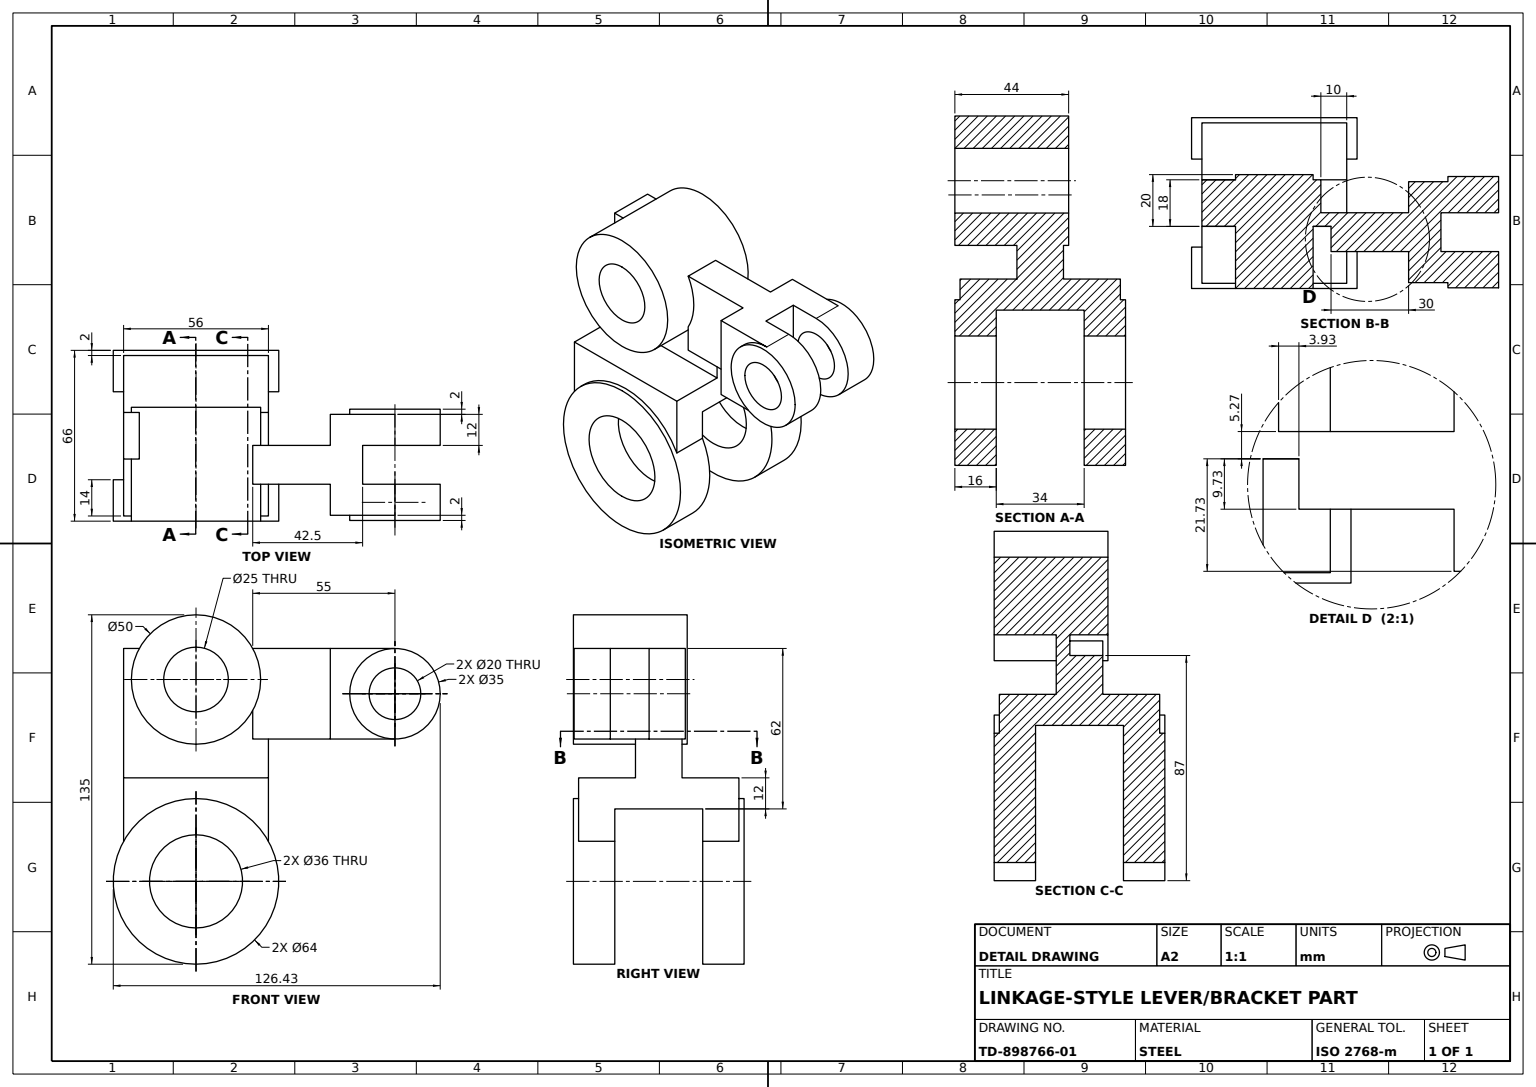
ISO-10303-21;
HEADER;
FILE_DESCRIPTION((''),'2;1');
FILE_NAME('','',(''),(''),'','','');
FILE_SCHEMA(('AUTOMOTIVE_DESIGN'));
ENDSEC;
DATA;
#1=APPLICATION_CONTEXT('');
#2=PRODUCT_CONTEXT('',#1,'mechanical');
#3=PRODUCT('','','',(#2));
#4=PRODUCT_DEFINITION_FORMATION('','',#3);
#5=PRODUCT_DEFINITION_CONTEXT('',#1,'design');
#6=PRODUCT_DEFINITION('','',#4,#5);
#7=PRODUCT_DEFINITION_SHAPE('','',#6);
#8=(LENGTH_UNIT()NAMED_UNIT(*)SI_UNIT(.MILLI.,.METRE.));
#9=(NAMED_UNIT(*)PLANE_ANGLE_UNIT()SI_UNIT($,.RADIAN.));
#10=(NAMED_UNIT(*)SI_UNIT($,.STERADIAN.)SOLID_ANGLE_UNIT());
#11=UNCERTAINTY_MEASURE_WITH_UNIT(LENGTH_MEASURE(1.E-05),#8,'distance_accuracy_value','');
#12=(GEOMETRIC_REPRESENTATION_CONTEXT(3)GLOBAL_UNCERTAINTY_ASSIGNED_CONTEXT((#11))GLOBAL_UNIT_ASSIGNED_CONTEXT((#8,#9,#10))REPRESENTATION_CONTEXT('',''));
#13=CARTESIAN_POINT('',(17.,-60.,-28.));
#14=VERTEX_POINT('',#13);
#15=CARTESIAN_POINT('',(17.,-12.508067,-56.));
#16=VERTEX_POINT('',#15);
#17=CARTESIAN_POINT('',(17.,-28.,-28.));
#18=DIRECTION('',(1.,0.,0.));
#19=DIRECTION('',(0.,1.,0.));
#20=AXIS2_PLACEMENT_3D('',#17,#18,#19);
#21=CIRCLE('',#20,32.);
#22=EDGE_CURVE('',#14,#16,#21,.T.);
#23=ORIENTED_EDGE('',*,*,#22,.T.);
#24=CARTESIAN_POINT('',(31.,-12.508067,-56.));
#25=VERTEX_POINT('',#24);
#26=DIRECTION('',(-1.,0.,0.));
#27=VECTOR('',#26,1000.);
#28=LINE('',#15,#27);
#29=EDGE_CURVE('',#25,#16,#28,.T.);
#30=ORIENTED_EDGE('',*,*,#29,.F.);
#31=CARTESIAN_POINT('',(31.,4.,-28.));
#32=VERTEX_POINT('',#31);
#33=CARTESIAN_POINT('',(31.,-28.,-28.));
#34=AXIS2_PLACEMENT_3D('',#33,#18,#19);
#35=CIRCLE('',#34,32.);
#36=EDGE_CURVE('',#25,#32,#35,.T.);
#37=ORIENTED_EDGE('',*,*,#36,.T.);
#38=CARTESIAN_POINT('',(33.,4.,-28.));
#39=VERTEX_POINT('',#38);
#40=CARTESIAN_POINT('',(17.,4.,-28.));
#41=VECTOR('',#18,1000.);
#42=LINE('',#40,#41);
#43=EDGE_CURVE('',#32,#39,#42,.T.);
#44=ORIENTED_EDGE('',*,*,#43,.T.);
#45=CARTESIAN_POINT('',(33.,-60.,-28.));
#46=VERTEX_POINT('',#45);
#47=CARTESIAN_POINT('',(33.,-28.,-28.));
#48=AXIS2_PLACEMENT_3D('',#47,#18,#19);
#49=CIRCLE('',#48,32.);
#50=EDGE_CURVE('',#46,#39,#49,.T.);
#51=ORIENTED_EDGE('',*,*,#50,.F.);
#52=LINE('',#13,#41);
#53=EDGE_CURVE('',#14,#46,#52,.T.);
#54=ORIENTED_EDGE('',*,*,#53,.F.);
#55=EDGE_LOOP('',(#23,#30,#37,#44,#51,#54));
#56=FACE_OUTER_BOUND('',#55,.T.);
#57=CYLINDRICAL_SURFACE('',#20,32.);
#58=ADVANCED_FACE('',(#56),#57,.T.);
#59=CARTESIAN_POINT('',(-17.,0.,0.));
#60=VERTEX_POINT('',#59);
#61=CARTESIAN_POINT('',(17.,0.,0.));
#62=VERTEX_POINT('',#61);
#63=CARTESIAN_POINT('',(0.,0.,0.));
#64=LINE('',#63,#41);
#65=EDGE_CURVE('',#60,#62,#64,.T.);
#66=ORIENTED_EDGE('',*,*,#65,.F.);
#67=CARTESIAN_POINT('',(-17.,0.,-56.));
#68=VERTEX_POINT('',#67);
#69=DIRECTION('',(0.,0.,1.));
#70=VECTOR('',#69,1000.);
#71=LINE('',#67,#70);
#72=EDGE_CURVE('',#68,#60,#71,.T.);
#73=ORIENTED_EDGE('',*,*,#72,.F.);
#74=CARTESIAN_POINT('',(17.,0.,-56.));
#75=VERTEX_POINT('',#74);
#76=CARTESIAN_POINT('',(0.,0.,-56.));
#77=LINE('',#76,#41);
#78=EDGE_CURVE('',#68,#75,#77,.T.);
#79=ORIENTED_EDGE('',*,*,#78,.T.);
#80=LINE('',#74,#70);
#81=EDGE_CURVE('',#75,#62,#80,.T.);
#82=ORIENTED_EDGE('',*,*,#81,.T.);
#83=EDGE_LOOP('',(#66,#73,#79,#82));
#84=FACE_OUTER_BOUND('',#83,.T.);
#85=DIRECTION('',(0.,-1.,0.));
#86=DIRECTION('',(0.,0.,-1.));
#87=AXIS2_PLACEMENT_3D('',#76,#85,#86);
#88=PLANE('',#87);
#89=ADVANCED_FACE('',(#84),#88,.T.);
#90=CARTESIAN_POINT('',(3.731987,27.,-104.931712));
#91=VERTEX_POINT('',#90);
#92=CARTESIAN_POINT('',(-8.268013,27.,-104.931712));
#93=VERTEX_POINT('',#92);
#94=LINE('',#92,#27);
#95=EDGE_CURVE('',#91,#93,#94,.T.);
#96=ORIENTED_EDGE('',*,*,#95,.F.);
#97=CARTESIAN_POINT('',(3.731987,27.,-92.431712));
#98=VERTEX_POINT('',#97);
#99=VECTOR('',#86,1000.);
#100=LINE('',#90,#99);
#101=EDGE_CURVE('',#98,#91,#100,.T.);
#102=ORIENTED_EDGE('',*,*,#101,.F.);
#103=CARTESIAN_POINT('',(18.731987,27.,-92.431712));
#104=VERTEX_POINT('',#103);
#105=LINE('',#97,#27);
#106=EDGE_CURVE('',#104,#98,#105,.T.);
#107=ORIENTED_EDGE('',*,*,#106,.F.);
#108=CARTESIAN_POINT('',(18.731987,27.,-104.931712));
#109=VERTEX_POINT('',#108);
#110=LINE('',#103,#70);
#111=EDGE_CURVE('',#109,#104,#110,.T.);
#112=ORIENTED_EDGE('',*,*,#111,.F.);
#113=CARTESIAN_POINT('',(30.731987,27.,-104.931712));
#114=VERTEX_POINT('',#113);
#115=LINE('',#108,#27);
#116=EDGE_CURVE('',#114,#109,#115,.T.);
#117=ORIENTED_EDGE('',*,*,#116,.F.);
#118=CARTESIAN_POINT('',(30.731987,27.,-79.931712));
#119=VERTEX_POINT('',#118);
#120=LINE('',#113,#99);
#121=EDGE_CURVE('',#119,#114,#120,.T.);
#122=ORIENTED_EDGE('',*,*,#121,.F.);
#123=CARTESIAN_POINT('',(18.731987,27.,-79.931712));
#124=VERTEX_POINT('',#123);
#125=LINE('',#118,#41);
#126=EDGE_CURVE('',#124,#119,#125,.T.);
#127=ORIENTED_EDGE('',*,*,#126,.F.);
#128=CARTESIAN_POINT('',(18.731987,27.,-49.931712));
#129=VERTEX_POINT('',#128);
#130=LINE('',#123,#99);
#131=EDGE_CURVE('',#129,#124,#130,.T.);
#132=ORIENTED_EDGE('',*,*,#131,.F.);
#133=CARTESIAN_POINT('',(9.,27.,-49.931712));
#134=VERTEX_POINT('',#133);
#135=CARTESIAN_POINT('',(3.731987,27.,-49.931712));
#136=LINE('',#135,#41);
#137=EDGE_CURVE('',#134,#129,#136,.T.);
#138=ORIENTED_EDGE('',*,*,#137,.F.);
#139=CARTESIAN_POINT('',(9.,27.,-56.));
#140=VERTEX_POINT('',#139);
#141=LINE('',#139,#99);
#142=EDGE_CURVE('',#134,#140,#141,.T.);
#143=ORIENTED_EDGE('',*,*,#142,.T.);
#144=CARTESIAN_POINT('',(3.731987,27.,-56.));
#145=VERTEX_POINT('',#144);
#146=CARTESIAN_POINT('',(0.,27.,-56.));
#147=LINE('',#146,#41);
#148=EDGE_CURVE('',#145,#140,#147,.T.);
#149=ORIENTED_EDGE('',*,*,#148,.F.);
#150=CARTESIAN_POINT('',(3.731987,27.,-79.931712));
#151=VERTEX_POINT('',#150);
#152=LINE('',#135,#70);
#153=EDGE_CURVE('',#151,#145,#152,.T.);
#154=ORIENTED_EDGE('',*,*,#153,.F.);
#155=CARTESIAN_POINT('',(-8.268013,27.,-79.931712));
#156=VERTEX_POINT('',#155);
#157=LINE('',#150,#41);
#158=EDGE_CURVE('',#156,#151,#157,.T.);
#159=ORIENTED_EDGE('',*,*,#158,.F.);
#160=LINE('',#155,#70);
#161=EDGE_CURVE('',#93,#156,#160,.T.);
#162=ORIENTED_EDGE('',*,*,#161,.F.);
#163=EDGE_LOOP('',(#96,#102,#107,#112,#117,#122,#127,#132,#138,#143,#149,#154,#159,#162));
#164=FACE_OUTER_BOUND('',#163,.T.);
#165=CARTESIAN_POINT('',(0.,27.,0.));
#166=AXIS2_PLACEMENT_3D('',#165,#85,#86);
#167=PLANE('',#166);
#168=ADVANCED_FACE('',(#164),#167,.T.);
#169=CARTESIAN_POINT('',(18.731987,38.,-49.931712));
#170=VERTEX_POINT('',#169);
#171=CARTESIAN_POINT('',(18.731987,62.,-49.931712));
#172=VERTEX_POINT('',#171);
#173=CARTESIAN_POINT('',(18.731987,50.,-28.));
#174=AXIS2_PLACEMENT_3D('',#173,#18,#86);
#175=CIRCLE('',#174,25.);
#176=EDGE_CURVE('',#170,#172,#175,.T.);
#177=ORIENTED_EDGE('',*,*,#176,.F.);
#178=VECTOR('',#19,1000.);
#179=LINE('',#128,#178);
#180=EDGE_CURVE('',#129,#170,#179,.T.);
#181=ORIENTED_EDGE('',*,*,#180,.F.);
#182=ORIENTED_EDGE('',*,*,#131,.T.);
#183=CARTESIAN_POINT('',(18.731987,62.,-79.931712));
#184=VERTEX_POINT('',#183);
#185=LINE('',#123,#178);
#186=EDGE_CURVE('',#124,#184,#185,.T.);
#187=ORIENTED_EDGE('',*,*,#186,.T.);
#188=LINE('',#183,#99);
#189=EDGE_CURVE('',#172,#184,#188,.T.);
#190=ORIENTED_EDGE('',*,*,#189,.F.);
#191=EDGE_LOOP('',(#177,#181,#182,#187,#190));
#192=FACE_OUTER_BOUND('',#191,.T.);
#193=AXIS2_PLACEMENT_3D('',#123,#18,#86);
#194=PLANE('',#193);
#195=ADVANCED_FACE('',(#192),#194,.T.);
#196=CARTESIAN_POINT('',(32.731987,44.5,-122.431712));
#197=VERTEX_POINT('',#196);
#198=CARTESIAN_POINT('',(18.731987,44.5,-122.431712));
#199=VERTEX_POINT('',#198);
#200=LINE('',#196,#27);
#201=EDGE_CURVE('',#197,#199,#200,.T.);
#202=ORIENTED_EDGE('',*,*,#201,.T.);
#203=CARTESIAN_POINT('',(18.731987,62.,-104.931712));
#204=VERTEX_POINT('',#203);
#205=CARTESIAN_POINT('',(18.731987,44.5,-104.931712));
#206=AXIS2_PLACEMENT_3D('',#205,#18,#86);
#207=CIRCLE('',#206,17.5);
#208=EDGE_CURVE('',#199,#204,#207,.T.);
#209=ORIENTED_EDGE('',*,*,#208,.T.);
#210=CARTESIAN_POINT('',(30.731987,62.,-104.931712));
#211=VERTEX_POINT('',#210);
#212=LINE('',#203,#27);
#213=EDGE_CURVE('',#211,#204,#212,.T.);
#214=ORIENTED_EDGE('',*,*,#213,.F.);
#215=CARTESIAN_POINT('',(30.731987,44.5,-87.431712));
#216=VERTEX_POINT('',#215);
#217=CARTESIAN_POINT('',(30.731987,44.5,-104.931712));
#218=AXIS2_PLACEMENT_3D('',#217,#18,#86);
#219=CIRCLE('',#218,17.5);
#220=EDGE_CURVE('',#211,#216,#219,.T.);
#221=ORIENTED_EDGE('',*,*,#220,.T.);
#222=CARTESIAN_POINT('',(32.731987,44.5,-87.431712));
#223=VERTEX_POINT('',#222);
#224=LINE('',#222,#27);
#225=EDGE_CURVE('',#223,#216,#224,.T.);
#226=ORIENTED_EDGE('',*,*,#225,.F.);
#227=CARTESIAN_POINT('',(32.731987,44.5,-104.931712));
#228=AXIS2_PLACEMENT_3D('',#227,#18,#86);
#229=CIRCLE('',#228,17.5);
#230=EDGE_CURVE('',#197,#223,#229,.T.);
#231=ORIENTED_EDGE('',*,*,#230,.F.);
#232=EDGE_LOOP('',(#202,#209,#214,#221,#226,#231));
#233=FACE_OUTER_BOUND('',#232,.T.);
#234=AXIS2_PLACEMENT_3D('',#227,#26,#69);
#235=CYLINDRICAL_SURFACE('',#234,17.5);
#236=ADVANCED_FACE('',(#233),#235,.T.);
#237=CARTESIAN_POINT('',(9.,62.,-6.068288));
#238=VERTEX_POINT('',#237);
#239=CARTESIAN_POINT('',(9.,25.,-28.));
#240=VERTEX_POINT('',#239);
#241=CARTESIAN_POINT('',(9.,50.,-28.));
#242=AXIS2_PLACEMENT_3D('',#241,#18,#19);
#243=CIRCLE('',#242,25.);
#244=EDGE_CURVE('',#238,#240,#243,.T.);
#245=ORIENTED_EDGE('',*,*,#244,.F.);
#246=CARTESIAN_POINT('',(9.,62.,0.));
#247=VERTEX_POINT('',#246);
#248=CARTESIAN_POINT('',(9.,62.,-56.));
#249=LINE('',#248,#70);
#250=EDGE_CURVE('',#238,#247,#249,.T.);
#251=ORIENTED_EDGE('',*,*,#250,.T.);
#252=CARTESIAN_POINT('',(9.,12.,0.));
#253=VERTEX_POINT('',#252);
#254=LINE('',#246,#178);
#255=EDGE_CURVE('',#253,#247,#254,.T.);
#256=ORIENTED_EDGE('',*,*,#255,.F.);
#257=CARTESIAN_POINT('',(9.,12.,-56.));
#258=VERTEX_POINT('',#257);
#259=LINE('',#257,#70);
#260=EDGE_CURVE('',#258,#253,#259,.T.);
#261=ORIENTED_EDGE('',*,*,#260,.F.);
#262=LINE('',#248,#178);
#263=EDGE_CURVE('',#258,#140,#262,.T.);
#264=ORIENTED_EDGE('',*,*,#263,.T.);
#265=ORIENTED_EDGE('',*,*,#142,.F.);
#266=CARTESIAN_POINT('',(9.,38.,-49.931712));
#267=VERTEX_POINT('',#266);
#268=CARTESIAN_POINT('',(9.,62.,-49.931712));
#269=VECTOR('',#85,1000.);
#270=LINE('',#268,#269);
#271=EDGE_CURVE('',#267,#134,#270,.T.);
#272=ORIENTED_EDGE('',*,*,#271,.F.);
#273=EDGE_CURVE('',#240,#267,#243,.T.);
#274=ORIENTED_EDGE('',*,*,#273,.F.);
#275=EDGE_LOOP('',(#245,#251,#256,#261,#264,#265,#272,#274));
#276=FACE_OUTER_BOUND('',#275,.T.);
#277=AXIS2_PLACEMENT_3D('',#248,#18,#19);
#278=PLANE('',#277);
#279=ADVANCED_FACE('',(#276),#278,.T.);
#280=CARTESIAN_POINT('',(-9.,27.,-56.));
#281=VERTEX_POINT('',#280);
#282=LINE('',#144,#27);
#283=EDGE_CURVE('',#145,#281,#282,.T.);
#284=ORIENTED_EDGE('',*,*,#283,.T.);
#285=CARTESIAN_POINT('',(-9.,27.,-46.));
#286=VERTEX_POINT('',#285);
#287=LINE('',#285,#99);
#288=EDGE_CURVE('',#286,#281,#287,.T.);
#289=ORIENTED_EDGE('',*,*,#288,.F.);
#290=CARTESIAN_POINT('',(3.731987,27.,-46.));
#291=VERTEX_POINT('',#290);
#292=LINE('',#290,#27);
#293=EDGE_CURVE('',#291,#286,#292,.T.);
#294=ORIENTED_EDGE('',*,*,#293,.F.);
#295=LINE('',#290,#99);
#296=EDGE_CURVE('',#291,#145,#295,.T.);
#297=ORIENTED_EDGE('',*,*,#296,.T.);
#298=EDGE_LOOP('',(#284,#289,#294,#297));
#299=FACE_OUTER_BOUND('',#298,.T.);
#300=AXIS2_PLACEMENT_3D('',#290,#85,#86);
#301=PLANE('',#300);
#302=ADVANCED_FACE('',(#299),#301,.F.);
#303=CARTESIAN_POINT('',(3.731987,62.,-104.931712));
#304=VERTEX_POINT('',#303);
#305=CARTESIAN_POINT('',(-8.268013,62.,-104.931712));
#306=VERTEX_POINT('',#305);
#307=LINE('',#305,#27);
#308=EDGE_CURVE('',#304,#306,#307,.T.);
#309=ORIENTED_EDGE('',*,*,#308,.T.);
#310=CARTESIAN_POINT('',(-8.268013,62.,-79.931712));
#311=VERTEX_POINT('',#310);
#312=LINE('',#310,#70);
#313=EDGE_CURVE('',#306,#311,#312,.T.);
#314=ORIENTED_EDGE('',*,*,#313,.T.);
#315=CARTESIAN_POINT('',(3.731987,62.,-79.931712));
#316=VERTEX_POINT('',#315);
#317=LINE('',#315,#41);
#318=EDGE_CURVE('',#311,#316,#317,.T.);
#319=ORIENTED_EDGE('',*,*,#318,.T.);
#320=CARTESIAN_POINT('',(3.731987,62.,-49.931712));
#321=VERTEX_POINT('',#320);
#322=LINE('',#320,#70);
#323=EDGE_CURVE('',#316,#321,#322,.T.);
#324=ORIENTED_EDGE('',*,*,#323,.T.);
#325=CARTESIAN_POINT('',(33.,62.,-49.931712));
#326=LINE('',#325,#27);
#327=EDGE_CURVE('',#172,#321,#326,.T.);
#328=ORIENTED_EDGE('',*,*,#327,.F.);
#329=ORIENTED_EDGE('',*,*,#189,.T.);
#330=CARTESIAN_POINT('',(30.731987,62.,-79.931712));
#331=VERTEX_POINT('',#330);
#332=LINE('',#330,#41);
#333=EDGE_CURVE('',#184,#331,#332,.T.);
#334=ORIENTED_EDGE('',*,*,#333,.T.);
#335=LINE('',#210,#99);
#336=EDGE_CURVE('',#331,#211,#335,.T.);
#337=ORIENTED_EDGE('',*,*,#336,.T.);
#338=ORIENTED_EDGE('',*,*,#213,.T.);
#339=CARTESIAN_POINT('',(18.731987,62.,-92.431712));
#340=VERTEX_POINT('',#339);
#341=LINE('',#339,#70);
#342=EDGE_CURVE('',#204,#340,#341,.T.);
#343=ORIENTED_EDGE('',*,*,#342,.T.);
#344=CARTESIAN_POINT('',(3.731987,62.,-92.431712));
#345=VERTEX_POINT('',#344);
#346=LINE('',#344,#27);
#347=EDGE_CURVE('',#340,#345,#346,.T.);
#348=ORIENTED_EDGE('',*,*,#347,.T.);
#349=LINE('',#303,#99);
#350=EDGE_CURVE('',#345,#304,#349,.T.);
#351=ORIENTED_EDGE('',*,*,#350,.T.);
#352=EDGE_LOOP('',(#309,#314,#319,#324,#328,#329,#334,#337,#338,#343,#348,#351));
#353=FACE_OUTER_BOUND('',#352,.T.);
#354=CARTESIAN_POINT('',(-9.,62.,-56.));
#355=AXIS2_PLACEMENT_3D('',#354,#19,#69);
#356=PLANE('',#355);
#357=ADVANCED_FACE('',(#353),#356,.T.);
#358=CARTESIAN_POINT('',(-33.,-28.,4.));
#359=VERTEX_POINT('',#358);
#360=CARTESIAN_POINT('',(-17.,-28.,4.));
#361=VERTEX_POINT('',#360);
#362=LINE('',#358,#41);
#363=EDGE_CURVE('',#359,#361,#362,.T.);
#364=ORIENTED_EDGE('',*,*,#363,.F.);
#365=CARTESIAN_POINT('',(-33.,-28.,-60.));
#366=VERTEX_POINT('',#365);
#367=CARTESIAN_POINT('',(-33.,-28.,-28.));
#368=AXIS2_PLACEMENT_3D('',#367,#26,#69);
#369=CIRCLE('',#368,32.);
#370=EDGE_CURVE('',#366,#359,#369,.T.);
#371=ORIENTED_EDGE('',*,*,#370,.F.);
#372=CARTESIAN_POINT('',(-17.,-28.,-60.));
#373=VERTEX_POINT('',#372);
#374=LINE('',#365,#41);
#375=EDGE_CURVE('',#366,#373,#374,.T.);
#376=ORIENTED_EDGE('',*,*,#375,.T.);
#377=CARTESIAN_POINT('',(-17.,-28.,-28.));
#378=AXIS2_PLACEMENT_3D('',#377,#18,#19);
#379=CIRCLE('',#378,32.);
#380=EDGE_CURVE('',#361,#373,#379,.T.);
#381=ORIENTED_EDGE('',*,*,#380,.F.);
#382=EDGE_LOOP('',(#364,#371,#376,#381));
#383=FACE_OUTER_BOUND('',#382,.T.);
#384=AXIS2_PLACEMENT_3D('',#367,#18,#86);
#385=CYLINDRICAL_SURFACE('',#384,32.);
#386=ADVANCED_FACE('',(#383),#385,.T.);
#387=CARTESIAN_POINT('',(17.,-12.508067,0.));
#388=VERTEX_POINT('',#387);
#389=LINE('',#61,#269);
#390=EDGE_CURVE('',#62,#388,#389,.T.);
#391=ORIENTED_EDGE('',*,*,#390,.T.);
#392=CARTESIAN_POINT('',(31.,-12.508067,0.));
#393=VERTEX_POINT('',#392);
#394=LINE('',#387,#27);
#395=EDGE_CURVE('',#393,#388,#394,.T.);
#396=ORIENTED_EDGE('',*,*,#395,.F.);
#397=CARTESIAN_POINT('',(31.,12.,0.));
#398=VERTEX_POINT('',#397);
#399=LINE('',#397,#178);
#400=EDGE_CURVE('',#393,#398,#399,.T.);
#401=ORIENTED_EDGE('',*,*,#400,.T.);
#402=LINE('',#252,#27);
#403=EDGE_CURVE('',#398,#253,#402,.T.);
#404=ORIENTED_EDGE('',*,*,#403,.T.);
#405=ORIENTED_EDGE('',*,*,#255,.T.);
#406=CARTESIAN_POINT('',(-9.,62.,0.));
#407=VERTEX_POINT('',#406);
#408=LINE('',#406,#27);
#409=EDGE_CURVE('',#247,#407,#408,.T.);
#410=ORIENTED_EDGE('',*,*,#409,.T.);
#411=CARTESIAN_POINT('',(-9.,12.,0.));
#412=VERTEX_POINT('',#411);
#413=LINE('',#406,#269);
#414=EDGE_CURVE('',#407,#412,#413,.T.);
#415=ORIENTED_EDGE('',*,*,#414,.T.);
#416=CARTESIAN_POINT('',(-31.,12.,0.));
#417=VERTEX_POINT('',#416);
#418=LINE('',#416,#27);
#419=EDGE_CURVE('',#412,#417,#418,.T.);
#420=ORIENTED_EDGE('',*,*,#419,.T.);
#421=CARTESIAN_POINT('',(-31.,-12.508067,0.));
#422=VERTEX_POINT('',#421);
#423=CARTESIAN_POINT('',(-31.,-48.,0.));
#424=LINE('',#423,#269);
#425=EDGE_CURVE('',#417,#422,#424,.T.);
#426=ORIENTED_EDGE('',*,*,#425,.T.);
#427=CARTESIAN_POINT('',(-17.,-12.508067,0.));
#428=VERTEX_POINT('',#427);
#429=LINE('',#421,#27);
#430=EDGE_CURVE('',#428,#422,#429,.T.);
#431=ORIENTED_EDGE('',*,*,#430,.F.);
#432=LINE('',#59,#178);
#433=EDGE_CURVE('',#428,#60,#432,.T.);
#434=ORIENTED_EDGE('',*,*,#433,.T.);
#435=ORIENTED_EDGE('',*,*,#65,.T.);
#436=EDGE_LOOP('',(#391,#396,#401,#404,#405,#410,#415,#420,#426,#431,#434,#435));
#437=FACE_OUTER_BOUND('',#436,.T.);
#438=AXIS2_PLACEMENT_3D('',#63,#69,#18);
#439=PLANE('',#438);
#440=ADVANCED_FACE('',(#437),#439,.T.);
#441=CARTESIAN_POINT('',(-11.,75.,-28.));
#442=VERTEX_POINT('',#441);
#443=CARTESIAN_POINT('',(-11.,25.,-28.));
#444=VERTEX_POINT('',#443);
#445=CARTESIAN_POINT('',(-11.,50.,-28.));
#446=AXIS2_PLACEMENT_3D('',#445,#26,#85);
#447=CIRCLE('',#446,25.);
#448=EDGE_CURVE('',#442,#444,#447,.T.);
#449=ORIENTED_EDGE('',*,*,#448,.T.);
#450=EDGE_CURVE('',#444,#442,#447,.T.);
#451=ORIENTED_EDGE('',*,*,#450,.T.);
#452=EDGE_LOOP('',(#449,#451));
#453=FACE_OUTER_BOUND('',#452,.T.);
#454=CARTESIAN_POINT('',(-11.,62.5,-28.));
#455=VERTEX_POINT('',#454);
#456=CARTESIAN_POINT('',(-11.,37.5,-28.));
#457=VERTEX_POINT('',#456);
#458=CIRCLE('',#446,12.5);
#459=EDGE_CURVE('',#455,#457,#458,.T.);
#460=ORIENTED_EDGE('',*,*,#459,.F.);
#461=EDGE_CURVE('',#457,#455,#458,.T.);
#462=ORIENTED_EDGE('',*,*,#461,.F.);
#463=EDGE_LOOP('',(#460,#462));
#464=FACE_BOUND('',#463,.T.);
#465=PLANE('',#446);
#466=ADVANCED_FACE('',(#453,#464),#465,.T.);
#467=CARTESIAN_POINT('',(32.731987,44.5,-94.931712));
#468=VERTEX_POINT('',#467);
#469=CARTESIAN_POINT('',(32.731987,44.5,-114.931712));
#470=VERTEX_POINT('',#469);
#471=CIRCLE('',#228,10.);
#472=EDGE_CURVE('',#468,#470,#471,.T.);
#473=ORIENTED_EDGE('',*,*,#472,.F.);
#474=EDGE_CURVE('',#470,#468,#471,.T.);
#475=ORIENTED_EDGE('',*,*,#474,.F.);
#476=EDGE_LOOP('',(#473,#475));
#477=FACE_BOUND('',#476,.T.);
#478=ORIENTED_EDGE('',*,*,#230,.T.);
#479=EDGE_CURVE('',#223,#197,#229,.T.);
#480=ORIENTED_EDGE('',*,*,#479,.T.);
#481=EDGE_LOOP('',(#478,#480));
#482=FACE_OUTER_BOUND('',#481,.T.);
#483=PLANE('',#228);
#484=ADVANCED_FACE('',(#477,#482),#483,.T.);
#485=LINE('',#118,#178);
#486=EDGE_CURVE('',#119,#331,#485,.T.);
#487=ORIENTED_EDGE('',*,*,#486,.F.);
#488=ORIENTED_EDGE('',*,*,#121,.T.);
#489=EDGE_CURVE('',#216,#114,#219,.T.);
#490=ORIENTED_EDGE('',*,*,#489,.F.);
#491=ORIENTED_EDGE('',*,*,#220,.F.);
#492=ORIENTED_EDGE('',*,*,#336,.F.);
#493=EDGE_LOOP('',(#487,#488,#490,#491,#492));
#494=FACE_OUTER_BOUND('',#493,.T.);
#495=AXIS2_PLACEMENT_3D('',#113,#18,#86);
#496=PLANE('',#495);
#497=ADVANCED_FACE('',(#494),#496,.T.);
#498=LINE('',#150,#178);
#499=EDGE_CURVE('',#151,#316,#498,.T.);
#500=ORIENTED_EDGE('',*,*,#499,.T.);
#501=ORIENTED_EDGE('',*,*,#318,.F.);
#502=LINE('',#155,#178);
#503=EDGE_CURVE('',#156,#311,#502,.T.);
#504=ORIENTED_EDGE('',*,*,#503,.F.);
#505=ORIENTED_EDGE('',*,*,#158,.T.);
#506=EDGE_LOOP('',(#500,#501,#504,#505));
#507=FACE_OUTER_BOUND('',#506,.T.);
#508=AXIS2_PLACEMENT_3D('',#150,#69,#18);
#509=PLANE('',#508);
#510=ADVANCED_FACE('',(#507),#509,.T.);
#511=EDGE_CURVE('',#32,#393,#35,.T.);
#512=ORIENTED_EDGE('',*,*,#511,.T.);
#513=ORIENTED_EDGE('',*,*,#395,.T.);
#514=EDGE_CURVE('',#388,#14,#21,.T.);
#515=ORIENTED_EDGE('',*,*,#514,.T.);
#516=ORIENTED_EDGE('',*,*,#53,.T.);
#517=EDGE_CURVE('',#39,#46,#49,.T.);
#518=ORIENTED_EDGE('',*,*,#517,.F.);
#519=ORIENTED_EDGE('',*,*,#43,.F.);
#520=EDGE_LOOP('',(#512,#513,#515,#516,#518,#519));
#521=FACE_OUTER_BOUND('',#520,.T.);
#522=ADVANCED_FACE('',(#521),#57,.T.);
#523=CARTESIAN_POINT('',(33.,62.5,-28.));
#524=VERTEX_POINT('',#523);
#525=LINE('',#454,#41);
#526=EDGE_CURVE('',#455,#524,#525,.T.);
#527=ORIENTED_EDGE('',*,*,#526,.F.);
#528=ORIENTED_EDGE('',*,*,#459,.T.);
#529=CARTESIAN_POINT('',(33.,37.5,-28.));
#530=VERTEX_POINT('',#529);
#531=LINE('',#456,#41);
#532=EDGE_CURVE('',#457,#530,#531,.T.);
#533=ORIENTED_EDGE('',*,*,#532,.T.);
#534=CARTESIAN_POINT('',(33.,50.,-28.));
#535=AXIS2_PLACEMENT_3D('',#534,#26,#85);
#536=CIRCLE('',#535,12.5);
#537=EDGE_CURVE('',#524,#530,#536,.T.);
#538=ORIENTED_EDGE('',*,*,#537,.F.);
#539=EDGE_LOOP('',(#527,#528,#533,#538));
#540=FACE_OUTER_BOUND('',#539,.T.);
#541=AXIS2_PLACEMENT_3D('',#445,#18,#19);
#542=CYLINDRICAL_SURFACE('',#541,12.5);
#543=ADVANCED_FACE('',(#540),#542,.F.);
#544=CARTESIAN_POINT('',(33.,75.,-28.));
#545=VERTEX_POINT('',#544);
#546=CARTESIAN_POINT('',(33.,25.,-28.));
#547=VERTEX_POINT('',#546);
#548=CIRCLE('',#535,25.);
#549=EDGE_CURVE('',#545,#547,#548,.T.);
#550=ORIENTED_EDGE('',*,*,#549,.F.);
#551=EDGE_CURVE('',#547,#545,#548,.T.);
#552=ORIENTED_EDGE('',*,*,#551,.F.);
#553=EDGE_LOOP('',(#550,#552));
#554=FACE_OUTER_BOUND('',#553,.T.);
#555=ORIENTED_EDGE('',*,*,#537,.T.);
#556=EDGE_CURVE('',#530,#524,#536,.T.);
#557=ORIENTED_EDGE('',*,*,#556,.T.);
#558=EDGE_LOOP('',(#555,#557));
#559=FACE_BOUND('',#558,.T.);
#560=PLANE('',#535);
#561=ADVANCED_FACE('',(#554,#559),#560,.F.);
#562=CARTESIAN_POINT('',(17.,-46.,-28.));
#563=VERTEX_POINT('',#562);
#564=CARTESIAN_POINT('',(17.,-10.,-28.));
#565=VERTEX_POINT('',#564);
#566=CIRCLE('',#20,18.);
#567=EDGE_CURVE('',#563,#565,#566,.T.);
#568=ORIENTED_EDGE('',*,*,#567,.T.);
#569=EDGE_CURVE('',#565,#563,#566,.T.);
#570=ORIENTED_EDGE('',*,*,#569,.T.);
#571=EDGE_LOOP('',(#568,#570));
#572=FACE_BOUND('',#571,.T.);
#573=LINE('',#74,#269);
#574=EDGE_CURVE('',#75,#16,#573,.T.);
#575=ORIENTED_EDGE('',*,*,#574,.T.);
#576=ORIENTED_EDGE('',*,*,#22,.F.);
#577=ORIENTED_EDGE('',*,*,#514,.F.);
#578=ORIENTED_EDGE('',*,*,#390,.F.);
#579=ORIENTED_EDGE('',*,*,#81,.F.);
#580=EDGE_LOOP('',(#575,#576,#577,#578,#579));
#581=FACE_OUTER_BOUND('',#580,.T.);
#582=AXIS2_PLACEMENT_3D('',#74,#26,#85);
#583=PLANE('',#582);
#584=ADVANCED_FACE('',(#572,#581),#583,.T.);
#585=CARTESIAN_POINT('',(3.731987,44.5,-114.931712));
#586=VERTEX_POINT('',#585);
#587=CARTESIAN_POINT('',(3.731987,44.5,-94.931712));
#588=VERTEX_POINT('',#587);
#589=CARTESIAN_POINT('',(3.731987,44.5,-104.931712));
#590=AXIS2_PLACEMENT_3D('',#589,#26,#69);
#591=CIRCLE('',#590,10.);
#592=EDGE_CURVE('',#586,#588,#591,.T.);
#593=ORIENTED_EDGE('',*,*,#592,.T.);
#594=EDGE_CURVE('',#588,#586,#591,.T.);
#595=ORIENTED_EDGE('',*,*,#594,.T.);
#596=EDGE_LOOP('',(#593,#595));
#597=FACE_BOUND('',#596,.T.);
#598=LINE('',#97,#178);
#599=EDGE_CURVE('',#98,#345,#598,.T.);
#600=ORIENTED_EDGE('',*,*,#599,.F.);
#601=ORIENTED_EDGE('',*,*,#101,.T.);
#602=CARTESIAN_POINT('',(3.731987,44.5,-122.431712));
#603=VERTEX_POINT('',#602);
#604=CIRCLE('',#590,17.5);
#605=EDGE_CURVE('',#603,#91,#604,.T.);
#606=ORIENTED_EDGE('',*,*,#605,.F.);
#607=EDGE_CURVE('',#304,#603,#604,.T.);
#608=ORIENTED_EDGE('',*,*,#607,.F.);
#609=ORIENTED_EDGE('',*,*,#350,.F.);
#610=EDGE_LOOP('',(#600,#601,#606,#608,#609));
#611=FACE_OUTER_BOUND('',#610,.T.);
#612=AXIS2_PLACEMENT_3D('',#90,#18,#86);
#613=PLANE('',#612);
#614=ADVANCED_FACE('',(#597,#611),#613,.T.);
#615=LINE('',#441,#41);
#616=EDGE_CURVE('',#442,#545,#615,.T.);
#617=ORIENTED_EDGE('',*,*,#616,.F.);
#618=ORIENTED_EDGE('',*,*,#450,.F.);
#619=CARTESIAN_POINT('',(-9.,25.,-28.));
#620=VERTEX_POINT('',#619);
#621=LINE('',#443,#41);
#622=EDGE_CURVE('',#444,#620,#621,.T.);
#623=ORIENTED_EDGE('',*,*,#622,.T.);
#624=CARTESIAN_POINT('',(-9.,62.,-6.068288));
#625=VERTEX_POINT('',#624);
#626=CARTESIAN_POINT('',(-9.,50.,-28.));
#627=AXIS2_PLACEMENT_3D('',#626,#26,#85);
#628=CIRCLE('',#627,25.);
#629=EDGE_CURVE('',#620,#625,#628,.T.);
#630=ORIENTED_EDGE('',*,*,#629,.T.);
#631=CARTESIAN_POINT('',(33.,62.,-6.068288));
#632=LINE('',#631,#41);
#633=EDGE_CURVE('',#625,#238,#632,.T.);
#634=ORIENTED_EDGE('',*,*,#633,.T.);
#635=ORIENTED_EDGE('',*,*,#244,.T.);
#636=EDGE_CURVE('',#240,#547,#621,.T.);
#637=ORIENTED_EDGE('',*,*,#636,.T.);
#638=ORIENTED_EDGE('',*,*,#551,.T.);
#639=EDGE_LOOP('',(#617,#618,#623,#630,#634,#635,#637,#638));
#640=FACE_OUTER_BOUND('',#639,.T.);
#641=CYLINDRICAL_SURFACE('',#541,25.);
#642=ADVANCED_FACE('',(#640),#641,.T.);
#643=ORIENTED_EDGE('',*,*,#363,.T.);
#644=EDGE_CURVE('',#428,#361,#379,.T.);
#645=ORIENTED_EDGE('',*,*,#644,.F.);
#646=ORIENTED_EDGE('',*,*,#430,.T.);
#647=CARTESIAN_POINT('',(-31.,-12.508067,-56.));
#648=VERTEX_POINT('',#647);
#649=CARTESIAN_POINT('',(-31.,-28.,-28.));
#650=AXIS2_PLACEMENT_3D('',#649,#26,#69);
#651=CIRCLE('',#650,32.);
#652=EDGE_CURVE('',#422,#648,#651,.T.);
#653=ORIENTED_EDGE('',*,*,#652,.T.);
#654=CARTESIAN_POINT('',(-17.,-12.508067,-56.));
#655=VERTEX_POINT('',#654);
#656=LINE('',#647,#27);
#657=EDGE_CURVE('',#655,#648,#656,.T.);
#658=ORIENTED_EDGE('',*,*,#657,.F.);
#659=EDGE_CURVE('',#373,#655,#379,.T.);
#660=ORIENTED_EDGE('',*,*,#659,.F.);
#661=ORIENTED_EDGE('',*,*,#375,.F.);
#662=EDGE_CURVE('',#359,#366,#369,.T.);
#663=ORIENTED_EDGE('',*,*,#662,.F.);
#664=EDGE_LOOP('',(#643,#645,#646,#653,#658,#660,#661,#663));
#665=FACE_OUTER_BOUND('',#664,.T.);
#666=ADVANCED_FACE('',(#665),#385,.T.);
#667=ORIENTED_EDGE('',*,*,#116,.T.);
#668=EDGE_CURVE('',#109,#199,#207,.T.);
#669=ORIENTED_EDGE('',*,*,#668,.T.);
#670=ORIENTED_EDGE('',*,*,#201,.F.);
#671=ORIENTED_EDGE('',*,*,#479,.F.);
#672=ORIENTED_EDGE('',*,*,#225,.T.);
#673=ORIENTED_EDGE('',*,*,#489,.T.);
#674=EDGE_LOOP('',(#667,#669,#670,#671,#672,#673));
#675=FACE_OUTER_BOUND('',#674,.T.);
#676=ADVANCED_FACE('',(#675),#235,.T.);
#677=ORIENTED_EDGE('',*,*,#419,.F.);
#678=CARTESIAN_POINT('',(-9.,12.,-56.));
#679=VERTEX_POINT('',#678);
#680=LINE('',#678,#70);
#681=EDGE_CURVE('',#679,#412,#680,.T.);
#682=ORIENTED_EDGE('',*,*,#681,.F.);
#683=CARTESIAN_POINT('',(-31.,12.,-56.));
#684=VERTEX_POINT('',#683);
#685=LINE('',#683,#27);
#686=EDGE_CURVE('',#679,#684,#685,.T.);
#687=ORIENTED_EDGE('',*,*,#686,.T.);
#688=LINE('',#683,#70);
#689=EDGE_CURVE('',#684,#417,#688,.T.);
#690=ORIENTED_EDGE('',*,*,#689,.T.);
#691=EDGE_LOOP('',(#677,#682,#687,#690));
#692=FACE_OUTER_BOUND('',#691,.T.);
#693=AXIS2_PLACEMENT_3D('',#683,#19,#26);
#694=PLANE('',#693);
#695=ADVANCED_FACE('',(#692),#694,.T.);
#696=CARTESIAN_POINT('',(-33.,-10.,-28.));
#697=VERTEX_POINT('',#696);
#698=CARTESIAN_POINT('',(-33.,-46.,-28.));
#699=VERTEX_POINT('',#698);
#700=CIRCLE('',#368,18.);
#701=EDGE_CURVE('',#697,#699,#700,.T.);
#702=ORIENTED_EDGE('',*,*,#701,.T.);
#703=CARTESIAN_POINT('',(-17.,-46.,-28.));
#704=VERTEX_POINT('',#703);
#705=CARTESIAN_POINT('',(-31.,-46.,-28.));
#706=LINE('',#705,#41);
#707=EDGE_CURVE('',#699,#704,#706,.T.);
#708=ORIENTED_EDGE('',*,*,#707,.T.);
#709=CARTESIAN_POINT('',(-17.,-10.,-28.));
#710=VERTEX_POINT('',#709);
#711=CIRCLE('',#378,18.);
#712=EDGE_CURVE('',#704,#710,#711,.T.);
#713=ORIENTED_EDGE('',*,*,#712,.T.);
#714=CARTESIAN_POINT('',(-31.,-10.,-28.));
#715=LINE('',#714,#41);
#716=EDGE_CURVE('',#697,#710,#715,.T.);
#717=ORIENTED_EDGE('',*,*,#716,.F.);
#718=EDGE_LOOP('',(#702,#708,#713,#717));
#719=FACE_OUTER_BOUND('',#718,.T.);
#720=AXIS2_PLACEMENT_3D('',#649,#18,#19);
#721=CYLINDRICAL_SURFACE('',#720,18.);
#722=ADVANCED_FACE('',(#719),#721,.F.);
#723=ORIENTED_EDGE('',*,*,#472,.T.);
#724=CARTESIAN_POINT('',(18.731987,44.5,-114.931712));
#725=VERTEX_POINT('',#724);
#726=CARTESIAN_POINT('',(33.,44.5,-114.931712));
#727=LINE('',#726,#27);
#728=EDGE_CURVE('',#470,#725,#727,.T.);
#729=ORIENTED_EDGE('',*,*,#728,.T.);
#730=CARTESIAN_POINT('',(18.731987,44.5,-94.931712));
#731=VERTEX_POINT('',#730);
#732=AXIS2_PLACEMENT_3D('',#205,#26,#69);
#733=CIRCLE('',#732,10.);
#734=EDGE_CURVE('',#725,#731,#733,.T.);
#735=ORIENTED_EDGE('',*,*,#734,.T.);
#736=CARTESIAN_POINT('',(33.,44.5,-94.931712));
#737=LINE('',#736,#27);
#738=EDGE_CURVE('',#468,#731,#737,.T.);
#739=ORIENTED_EDGE('',*,*,#738,.F.);
#740=EDGE_LOOP('',(#723,#729,#735,#739));
#741=FACE_OUTER_BOUND('',#740,.T.);
#742=CARTESIAN_POINT('',(33.,44.5,-104.931712));
#743=AXIS2_PLACEMENT_3D('',#742,#26,#69);
#744=CYLINDRICAL_SURFACE('',#743,10.);
#745=ADVANCED_FACE('',(#741),#744,.F.);
#746=CARTESIAN_POINT('',(-8.268013,44.5,-87.431712));
#747=VERTEX_POINT('',#746);
#748=CARTESIAN_POINT('',(-8.268013,44.5,-104.931712));
#749=AXIS2_PLACEMENT_3D('',#748,#26,#69);
#750=CIRCLE('',#749,17.5);
#751=EDGE_CURVE('',#747,#306,#750,.T.);
#752=ORIENTED_EDGE('',*,*,#751,.F.);
#753=EDGE_CURVE('',#93,#747,#750,.T.);
#754=ORIENTED_EDGE('',*,*,#753,.F.);
#755=ORIENTED_EDGE('',*,*,#161,.T.);
#756=ORIENTED_EDGE('',*,*,#503,.T.);
#757=ORIENTED_EDGE('',*,*,#313,.F.);
#758=EDGE_LOOP('',(#752,#754,#755,#756,#757));
#759=FACE_OUTER_BOUND('',#758,.T.);
#760=AXIS2_PLACEMENT_3D('',#155,#26,#69);
#761=PLANE('',#760);
#762=ADVANCED_FACE('',(#759),#761,.T.);
#763=ORIENTED_EDGE('',*,*,#461,.T.);
#764=ORIENTED_EDGE('',*,*,#526,.T.);
#765=ORIENTED_EDGE('',*,*,#556,.F.);
#766=ORIENTED_EDGE('',*,*,#532,.F.);
#767=EDGE_LOOP('',(#763,#764,#765,#766));
#768=FACE_OUTER_BOUND('',#767,.T.);
#769=ADVANCED_FACE('',(#768),#542,.F.);
#770=ORIENTED_EDGE('',*,*,#448,.F.);
#771=ORIENTED_EDGE('',*,*,#616,.T.);
#772=ORIENTED_EDGE('',*,*,#549,.T.);
#773=ORIENTED_EDGE('',*,*,#636,.F.);
#774=ORIENTED_EDGE('',*,*,#273,.T.);
#775=CARTESIAN_POINT('',(-11.,38.,-49.931712));
#776=LINE('',#775,#41);
#777=EDGE_CURVE('',#267,#170,#776,.T.);
#778=ORIENTED_EDGE('',*,*,#777,.T.);
#779=ORIENTED_EDGE('',*,*,#176,.T.);
#780=ORIENTED_EDGE('',*,*,#327,.T.);
#781=CARTESIAN_POINT('',(3.731987,32.650648,-46.));
#782=VERTEX_POINT('',#781);
#783=CARTESIAN_POINT('',(3.731987,50.,-28.));
#784=AXIS2_PLACEMENT_3D('',#783,#26,#69);
#785=CIRCLE('',#784,25.);
#786=EDGE_CURVE('',#321,#782,#785,.T.);
#787=ORIENTED_EDGE('',*,*,#786,.T.);
#788=CARTESIAN_POINT('',(-9.,32.650648,-46.));
#789=VERTEX_POINT('',#788);
#790=CARTESIAN_POINT('',(5.,32.650648,-46.));
#791=LINE('',#790,#27);
#792=EDGE_CURVE('',#782,#789,#791,.T.);
#793=ORIENTED_EDGE('',*,*,#792,.T.);
#794=EDGE_CURVE('',#789,#620,#628,.T.);
#795=ORIENTED_EDGE('',*,*,#794,.T.);
#796=ORIENTED_EDGE('',*,*,#622,.F.);
#797=EDGE_LOOP('',(#770,#771,#772,#773,#774,#778,#779,#780,#787,#793,#795,#796));
#798=FACE_OUTER_BOUND('',#797,.T.);
#799=ADVANCED_FACE('',(#798),#641,.T.);
#800=EDGE_CURVE('',#699,#697,#700,.T.);
#801=ORIENTED_EDGE('',*,*,#800,.T.);
#802=ORIENTED_EDGE('',*,*,#716,.T.);
#803=EDGE_CURVE('',#710,#704,#711,.T.);
#804=ORIENTED_EDGE('',*,*,#803,.T.);
#805=ORIENTED_EDGE('',*,*,#707,.F.);
#806=EDGE_LOOP('',(#801,#802,#804,#805));
#807=FACE_OUTER_BOUND('',#806,.T.);
#808=ADVANCED_FACE('',(#807),#721,.F.);
#809=CARTESIAN_POINT('',(-10.268013,44.5,-114.931712));
#810=VERTEX_POINT('',#809);
#811=LINE('',#809,#41);
#812=EDGE_CURVE('',#810,#586,#811,.T.);
#813=ORIENTED_EDGE('',*,*,#812,.F.);
#814=CARTESIAN_POINT('',(-10.268013,44.5,-94.931712));
#815=VERTEX_POINT('',#814);
#816=CARTESIAN_POINT('',(-10.268013,44.5,-104.931712));
#817=AXIS2_PLACEMENT_3D('',#816,#26,#69);
#818=CIRCLE('',#817,10.);
#819=EDGE_CURVE('',#810,#815,#818,.T.);
#820=ORIENTED_EDGE('',*,*,#819,.T.);
#821=LINE('',#814,#41);
#822=EDGE_CURVE('',#815,#588,#821,.T.);
#823=ORIENTED_EDGE('',*,*,#822,.T.);
#824=ORIENTED_EDGE('',*,*,#592,.F.);
#825=EDGE_LOOP('',(#813,#820,#823,#824));
#826=FACE_OUTER_BOUND('',#825,.T.);
#827=AXIS2_PLACEMENT_3D('',#816,#18,#86);
#828=CYLINDRICAL_SURFACE('',#827,10.);
#829=ADVANCED_FACE('',(#826),#828,.F.);
#830=EDGE_CURVE('',#815,#810,#818,.T.);
#831=ORIENTED_EDGE('',*,*,#830,.T.);
#832=ORIENTED_EDGE('',*,*,#812,.T.);
#833=ORIENTED_EDGE('',*,*,#594,.F.);
#834=ORIENTED_EDGE('',*,*,#822,.F.);
#835=EDGE_LOOP('',(#831,#832,#833,#834));
#836=FACE_OUTER_BOUND('',#835,.T.);
#837=ADVANCED_FACE('',(#836),#828,.F.);
#838=ORIENTED_EDGE('',*,*,#499,.F.);
#839=ORIENTED_EDGE('',*,*,#153,.T.);
#840=ORIENTED_EDGE('',*,*,#296,.F.);
#841=CARTESIAN_POINT('',(3.731987,62.,-46.));
#842=LINE('',#841,#269);
#843=EDGE_CURVE('',#782,#291,#842,.T.);
#844=ORIENTED_EDGE('',*,*,#843,.F.);
#845=ORIENTED_EDGE('',*,*,#786,.F.);
#846=ORIENTED_EDGE('',*,*,#323,.F.);
#847=EDGE_LOOP('',(#838,#839,#840,#844,#845,#846));
#848=FACE_OUTER_BOUND('',#847,.T.);
#849=AXIS2_PLACEMENT_3D('',#135,#26,#69);
#850=PLANE('',#849);
#851=ADVANCED_FACE('',(#848),#850,.T.);
#852=ORIENTED_EDGE('',*,*,#486,.T.);
#853=ORIENTED_EDGE('',*,*,#333,.F.);
#854=ORIENTED_EDGE('',*,*,#186,.F.);
#855=ORIENTED_EDGE('',*,*,#126,.T.);
#856=EDGE_LOOP('',(#852,#853,#854,#855));
#857=FACE_OUTER_BOUND('',#856,.T.);
#858=AXIS2_PLACEMENT_3D('',#118,#69,#18);
#859=PLANE('',#858);
#860=ADVANCED_FACE('',(#857),#859,.T.);
#861=CARTESIAN_POINT('',(33.,-46.,-28.));
#862=VERTEX_POINT('',#861);
#863=CARTESIAN_POINT('',(33.,-10.,-28.));
#864=VERTEX_POINT('',#863);
#865=CIRCLE('',#48,18.);
#866=EDGE_CURVE('',#862,#864,#865,.T.);
#867=ORIENTED_EDGE('',*,*,#866,.F.);
#868=EDGE_CURVE('',#864,#862,#865,.T.);
#869=ORIENTED_EDGE('',*,*,#868,.F.);
#870=EDGE_LOOP('',(#867,#869));
#871=FACE_BOUND('',#870,.T.);
#872=ORIENTED_EDGE('',*,*,#517,.T.);
#873=ORIENTED_EDGE('',*,*,#50,.T.);
#874=EDGE_LOOP('',(#872,#873));
#875=FACE_OUTER_BOUND('',#874,.T.);
#876=PLANE('',#48);
#877=ADVANCED_FACE('',(#871,#875),#876,.T.);
#878=ORIENTED_EDGE('',*,*,#753,.T.);
#879=CARTESIAN_POINT('',(-10.268013,44.5,-87.431712));
#880=VERTEX_POINT('',#879);
#881=LINE('',#879,#41);
#882=EDGE_CURVE('',#880,#747,#881,.T.);
#883=ORIENTED_EDGE('',*,*,#882,.F.);
#884=CARTESIAN_POINT('',(-10.268013,44.5,-122.431712));
#885=VERTEX_POINT('',#884);
#886=CIRCLE('',#817,17.5);
#887=EDGE_CURVE('',#885,#880,#886,.T.);
#888=ORIENTED_EDGE('',*,*,#887,.F.);
#889=LINE('',#884,#41);
#890=EDGE_CURVE('',#885,#603,#889,.T.);
#891=ORIENTED_EDGE('',*,*,#890,.T.);
#892=ORIENTED_EDGE('',*,*,#605,.T.);
#893=ORIENTED_EDGE('',*,*,#95,.T.);
#894=EDGE_LOOP('',(#878,#883,#888,#891,#892,#893));
#895=FACE_OUTER_BOUND('',#894,.T.);
#896=CYLINDRICAL_SURFACE('',#827,17.5);
#897=ADVANCED_FACE('',(#895),#896,.T.);
#898=ORIENTED_EDGE('',*,*,#777,.F.);
#899=ORIENTED_EDGE('',*,*,#271,.T.);
#900=ORIENTED_EDGE('',*,*,#137,.T.);
#901=ORIENTED_EDGE('',*,*,#180,.T.);
#902=EDGE_LOOP('',(#898,#899,#900,#901));
#903=FACE_OUTER_BOUND('',#902,.T.);
#904=AXIS2_PLACEMENT_3D('',#135,#69,#18);
#905=PLANE('',#904);
#906=ADVANCED_FACE('',(#903),#905,.T.);
#907=CARTESIAN_POINT('',(31.,12.,-56.));
#908=VERTEX_POINT('',#907);
#909=LINE('',#907,#70);
#910=EDGE_CURVE('',#908,#398,#909,.T.);
#911=ORIENTED_EDGE('',*,*,#910,.T.);
#912=ORIENTED_EDGE('',*,*,#400,.F.);
#913=ORIENTED_EDGE('',*,*,#511,.F.);
#914=ORIENTED_EDGE('',*,*,#36,.F.);
#915=LINE('',#907,#178);
#916=EDGE_CURVE('',#25,#908,#915,.T.);
#917=ORIENTED_EDGE('',*,*,#916,.T.);
#918=EDGE_LOOP('',(#911,#912,#913,#914,#917));
#919=FACE_OUTER_BOUND('',#918,.T.);
#920=AXIS2_PLACEMENT_3D('',#907,#18,#19);
#921=PLANE('',#920);
#922=ADVANCED_FACE('',(#919),#921,.T.);
#923=ORIENTED_EDGE('',*,*,#803,.F.);
#924=ORIENTED_EDGE('',*,*,#712,.F.);
#925=EDGE_LOOP('',(#923,#924));
#926=FACE_BOUND('',#925,.T.);
#927=ORIENTED_EDGE('',*,*,#380,.T.);
#928=ORIENTED_EDGE('',*,*,#659,.T.);
#929=LINE('',#67,#178);
#930=EDGE_CURVE('',#655,#68,#929,.T.);
#931=ORIENTED_EDGE('',*,*,#930,.T.);
#932=ORIENTED_EDGE('',*,*,#72,.T.);
#933=ORIENTED_EDGE('',*,*,#433,.F.);
#934=ORIENTED_EDGE('',*,*,#644,.T.);
#935=EDGE_LOOP('',(#927,#928,#931,#932,#933,#934));
#936=FACE_OUTER_BOUND('',#935,.T.);
#937=AXIS2_PLACEMENT_3D('',#67,#18,#19);
#938=PLANE('',#937);
#939=ADVANCED_FACE('',(#926,#936),#938,.T.);
#940=LINE('',#564,#41);
#941=EDGE_CURVE('',#565,#864,#940,.T.);
#942=ORIENTED_EDGE('',*,*,#941,.F.);
#943=ORIENTED_EDGE('',*,*,#567,.F.);
#944=LINE('',#562,#41);
#945=EDGE_CURVE('',#563,#862,#944,.T.);
#946=ORIENTED_EDGE('',*,*,#945,.T.);
#947=ORIENTED_EDGE('',*,*,#866,.T.);
#948=EDGE_LOOP('',(#942,#943,#946,#947));
#949=FACE_OUTER_BOUND('',#948,.T.);
#950=CYLINDRICAL_SURFACE('',#20,18.);
#951=ADVANCED_FACE('',(#949),#950,.F.);
#952=LINE('',#354,#70);
#953=EDGE_CURVE('',#625,#407,#952,.T.);
#954=ORIENTED_EDGE('',*,*,#953,.T.);
#955=ORIENTED_EDGE('',*,*,#409,.F.);
#956=ORIENTED_EDGE('',*,*,#250,.F.);
#957=ORIENTED_EDGE('',*,*,#633,.F.);
#958=EDGE_LOOP('',(#954,#955,#956,#957));
#959=FACE_OUTER_BOUND('',#958,.T.);
#960=ADVANCED_FACE('',(#959),#356,.T.);
#961=ORIENTED_EDGE('',*,*,#728,.F.);
#962=ORIENTED_EDGE('',*,*,#474,.T.);
#963=ORIENTED_EDGE('',*,*,#738,.T.);
#964=EDGE_CURVE('',#731,#725,#733,.T.);
#965=ORIENTED_EDGE('',*,*,#964,.T.);
#966=EDGE_LOOP('',(#961,#962,#963,#965));
#967=FACE_OUTER_BOUND('',#966,.T.);
#968=ADVANCED_FACE('',(#967),#744,.F.);
#969=ORIENTED_EDGE('',*,*,#293,.T.);
#970=LINE('',#285,#178);
#971=EDGE_CURVE('',#286,#789,#970,.T.);
#972=ORIENTED_EDGE('',*,*,#971,.T.);
#973=ORIENTED_EDGE('',*,*,#792,.F.);
#974=ORIENTED_EDGE('',*,*,#843,.T.);
#975=EDGE_LOOP('',(#969,#972,#973,#974));
#976=FACE_OUTER_BOUND('',#975,.T.);
#977=CARTESIAN_POINT('',(0.,0.,-46.));
#978=AXIS2_PLACEMENT_3D('',#977,#86,#26);
#979=PLANE('',#978);
#980=ADVANCED_FACE('',(#976),#979,.T.);
#981=ORIENTED_EDGE('',*,*,#629,.F.);
#982=ORIENTED_EDGE('',*,*,#794,.F.);
#983=ORIENTED_EDGE('',*,*,#971,.F.);
#984=ORIENTED_EDGE('',*,*,#288,.T.);
#985=LINE('',#354,#269);
#986=EDGE_CURVE('',#281,#679,#985,.T.);
#987=ORIENTED_EDGE('',*,*,#986,.T.);
#988=ORIENTED_EDGE('',*,*,#681,.T.);
#989=ORIENTED_EDGE('',*,*,#414,.F.);
#990=ORIENTED_EDGE('',*,*,#953,.F.);
#991=EDGE_LOOP('',(#981,#982,#983,#984,#987,#988,#989,#990));
#992=FACE_OUTER_BOUND('',#991,.T.);
#993=AXIS2_PLACEMENT_3D('',#354,#26,#85);
#994=PLANE('',#993);
#995=ADVANCED_FACE('',(#992),#994,.T.);
#996=CARTESIAN_POINT('',(-31.,-48.,-56.));
#997=LINE('',#996,#269);
#998=EDGE_CURVE('',#684,#648,#997,.T.);
#999=ORIENTED_EDGE('',*,*,#998,.T.);
#1000=ORIENTED_EDGE('',*,*,#652,.F.);
#1001=ORIENTED_EDGE('',*,*,#425,.F.);
#1002=ORIENTED_EDGE('',*,*,#689,.F.);
#1003=EDGE_LOOP('',(#999,#1000,#1001,#1002));
#1004=FACE_OUTER_BOUND('',#1003,.T.);
#1005=AXIS2_PLACEMENT_3D('',#996,#26,#69);
#1006=PLANE('',#1005);
#1007=ADVANCED_FACE('',(#1004),#1006,.T.);
#1008=ORIENTED_EDGE('',*,*,#403,.F.);
#1009=ORIENTED_EDGE('',*,*,#910,.F.);
#1010=LINE('',#257,#27);
#1011=EDGE_CURVE('',#908,#258,#1010,.T.);
#1012=ORIENTED_EDGE('',*,*,#1011,.T.);
#1013=ORIENTED_EDGE('',*,*,#260,.T.);
#1014=EDGE_LOOP('',(#1008,#1009,#1012,#1013));
#1015=FACE_OUTER_BOUND('',#1014,.T.);
#1016=AXIS2_PLACEMENT_3D('',#257,#19,#26);
#1017=PLANE('',#1016);
#1018=ADVANCED_FACE('',(#1015),#1017,.T.);
#1019=ORIENTED_EDGE('',*,*,#887,.T.);
#1020=EDGE_CURVE('',#880,#885,#886,.T.);
#1021=ORIENTED_EDGE('',*,*,#1020,.T.);
#1022=EDGE_LOOP('',(#1019,#1021));
#1023=FACE_OUTER_BOUND('',#1022,.T.);
#1024=ORIENTED_EDGE('',*,*,#830,.F.);
#1025=ORIENTED_EDGE('',*,*,#819,.F.);
#1026=EDGE_LOOP('',(#1024,#1025));
#1027=FACE_BOUND('',#1026,.T.);
#1028=PLANE('',#817);
#1029=ADVANCED_FACE('',(#1023,#1027),#1028,.T.);
#1030=ORIENTED_EDGE('',*,*,#607,.T.);
#1031=ORIENTED_EDGE('',*,*,#890,.F.);
#1032=ORIENTED_EDGE('',*,*,#1020,.F.);
#1033=ORIENTED_EDGE('',*,*,#882,.T.);
#1034=ORIENTED_EDGE('',*,*,#751,.T.);
#1035=ORIENTED_EDGE('',*,*,#308,.F.);
#1036=EDGE_LOOP('',(#1030,#1031,#1032,#1033,#1034,#1035));
#1037=FACE_OUTER_BOUND('',#1036,.T.);
#1038=ADVANCED_FACE('',(#1037),#896,.T.);
#1039=ORIENTED_EDGE('',*,*,#342,.F.);
#1040=ORIENTED_EDGE('',*,*,#208,.F.);
#1041=ORIENTED_EDGE('',*,*,#668,.F.);
#1042=ORIENTED_EDGE('',*,*,#111,.T.);
#1043=LINE('',#103,#178);
#1044=EDGE_CURVE('',#104,#340,#1043,.T.);
#1045=ORIENTED_EDGE('',*,*,#1044,.T.);
#1046=EDGE_LOOP('',(#1039,#1040,#1041,#1042,#1045));
#1047=FACE_OUTER_BOUND('',#1046,.T.);
#1048=ORIENTED_EDGE('',*,*,#734,.F.);
#1049=ORIENTED_EDGE('',*,*,#964,.F.);
#1050=EDGE_LOOP('',(#1048,#1049));
#1051=FACE_BOUND('',#1050,.T.);
#1052=AXIS2_PLACEMENT_3D('',#103,#26,#69);
#1053=PLANE('',#1052);
#1054=ADVANCED_FACE('',(#1047,#1051),#1053,.T.);
#1055=ORIENTED_EDGE('',*,*,#686,.F.);
#1056=ORIENTED_EDGE('',*,*,#986,.F.);
#1057=ORIENTED_EDGE('',*,*,#283,.F.);
#1058=ORIENTED_EDGE('',*,*,#148,.T.);
#1059=ORIENTED_EDGE('',*,*,#263,.F.);
#1060=ORIENTED_EDGE('',*,*,#1011,.F.);
#1061=ORIENTED_EDGE('',*,*,#916,.F.);
#1062=ORIENTED_EDGE('',*,*,#29,.T.);
#1063=ORIENTED_EDGE('',*,*,#574,.F.);
#1064=ORIENTED_EDGE('',*,*,#78,.F.);
#1065=ORIENTED_EDGE('',*,*,#930,.F.);
#1066=ORIENTED_EDGE('',*,*,#657,.T.);
#1067=ORIENTED_EDGE('',*,*,#998,.F.);
#1068=EDGE_LOOP('',(#1055,#1056,#1057,#1058,#1059,#1060,#1061,#1062,#1063,#1064,#1065,#1066,#1067));
#1069=FACE_OUTER_BOUND('',#1068,.T.);
#1070=AXIS2_PLACEMENT_3D('',#76,#69,#18);
#1071=PLANE('',#1070);
#1072=ADVANCED_FACE('',(#1069),#1071,.F.);
#1073=ORIENTED_EDGE('',*,*,#347,.F.);
#1074=ORIENTED_EDGE('',*,*,#1044,.F.);
#1075=ORIENTED_EDGE('',*,*,#106,.T.);
#1076=ORIENTED_EDGE('',*,*,#599,.T.);
#1077=EDGE_LOOP('',(#1073,#1074,#1075,#1076));
#1078=FACE_OUTER_BOUND('',#1077,.T.);
#1079=AXIS2_PLACEMENT_3D('',#97,#86,#26);
#1080=PLANE('',#1079);
#1081=ADVANCED_FACE('',(#1078),#1080,.T.);
#1082=ORIENTED_EDGE('',*,*,#941,.T.);
#1083=ORIENTED_EDGE('',*,*,#868,.T.);
#1084=ORIENTED_EDGE('',*,*,#945,.F.);
#1085=ORIENTED_EDGE('',*,*,#569,.F.);
#1086=EDGE_LOOP('',(#1082,#1083,#1084,#1085));
#1087=FACE_OUTER_BOUND('',#1086,.T.);
#1088=ADVANCED_FACE('',(#1087),#950,.F.);
#1089=ORIENTED_EDGE('',*,*,#370,.T.);
#1090=ORIENTED_EDGE('',*,*,#662,.T.);
#1091=EDGE_LOOP('',(#1089,#1090));
#1092=FACE_OUTER_BOUND('',#1091,.T.);
#1093=ORIENTED_EDGE('',*,*,#701,.F.);
#1094=ORIENTED_EDGE('',*,*,#800,.F.);
#1095=EDGE_LOOP('',(#1093,#1094));
#1096=FACE_BOUND('',#1095,.T.);
#1097=PLANE('',#368);
#1098=ADVANCED_FACE('',(#1092,#1096),#1097,.T.);
#1099=CLOSED_SHELL('',(#58,#89,#168,#195,#236,#279,#302,#357,#386,#440,#466,#484,#497,#510,#522,#543,#561,#584,#614,#642,#666,#676,#695,#722,#745,#762,#769,#799,#808,#829,#837,#851,#860,#877,#897,#906,#922,#939,#951,#960,#968,#980,#995,#1007,#1018,#1029,#1038,#1054,#1072,#1081,#1088,#1098));
#1100=MANIFOLD_SOLID_BREP('',#1099);
#1101=ADVANCED_BREP_SHAPE_REPRESENTATION('',(#1100),#12);
#1102=SHAPE_DEFINITION_REPRESENTATION(#7,#1101);
ENDSEC;
END-ISO-10303-21;
